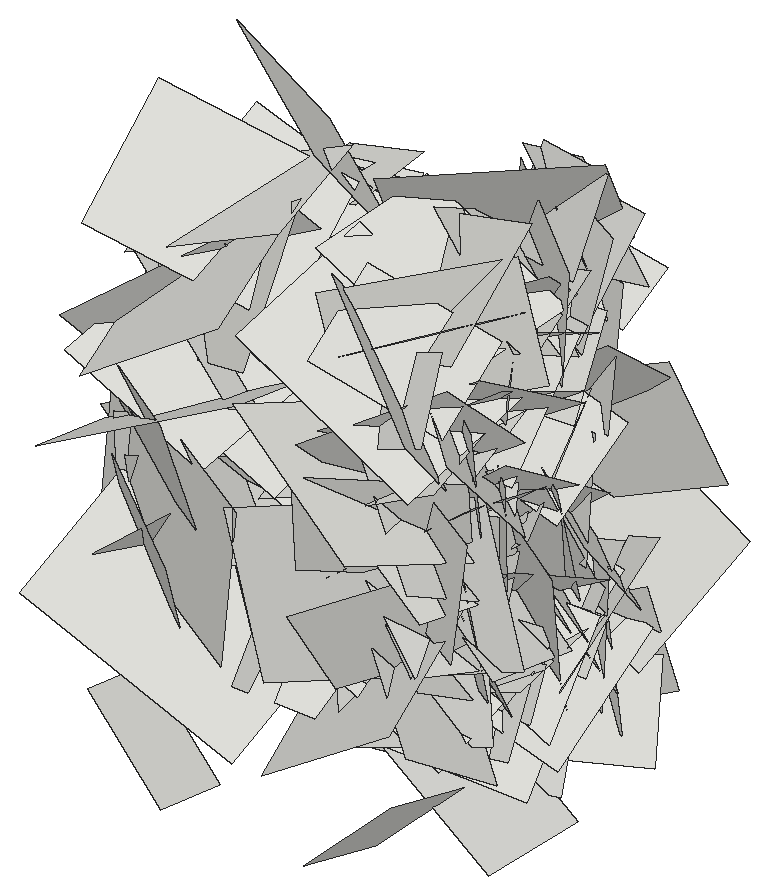
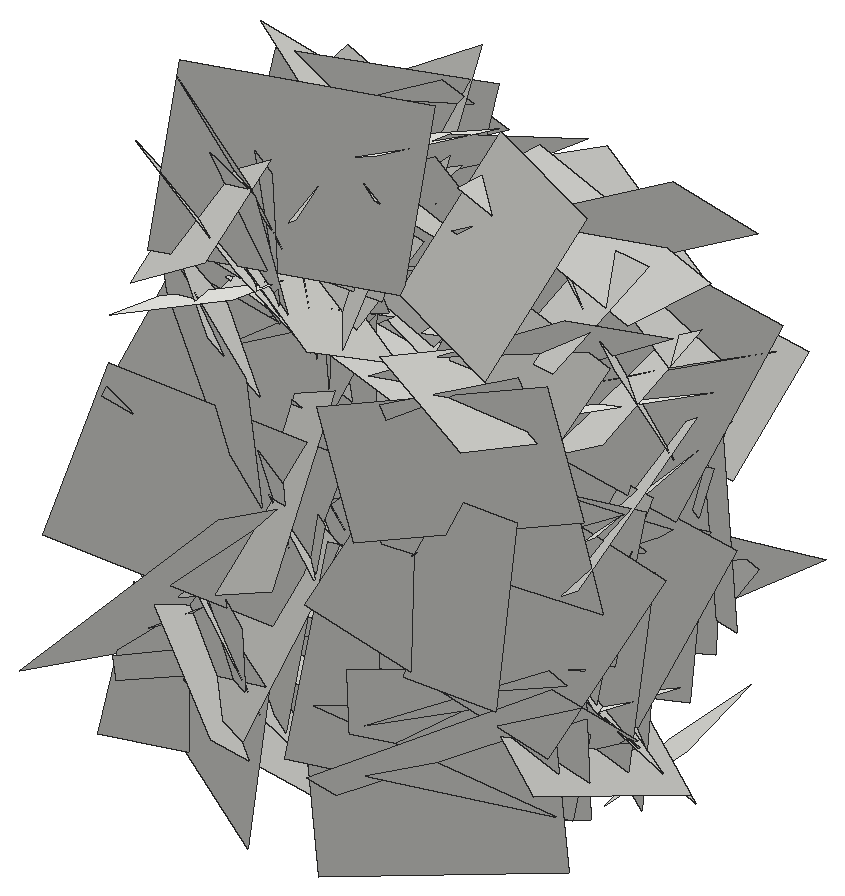
# SketchUp Ruby script. Lengths in inches.
U = 1.inch
M = Sketchup.active_model
def pt(a) = Geom::Point3d.new(a.map { |v| v * U })
def face(e, loops, mat)
  f = e.add_face(loops[0].map { |a| pt(a) })
  loops[1..].each { |l| e.add_face(l.map { |a| pt(a) }).erase! }
  f.material = f.back_material = mat if mat
  f
end
# faces: each face lists its corners as indices into pts; further lists are holes
def faces(e, pts, list, mat = nil) = list.each { |f| face(e, (f[0].is_a?(Array) ? f : [f]).map { |l| l.map { |i| pts[i] } }, mat) }
# xy, xz, yz: faces in a plane at the given z, y or x. An outline is a flat list of corners, or four numbers for a rectangle; further outlines are holes
def ring(l) = l.size == 4 ? [[l[0], l[1]], [l[2], l[1]], [l[2], l[3]], [l[0], l[3]]] : l.each_slice(2).to_a
def flat(e, list, mat, &to3) = list.each { |f| face(e, (f[0].is_a?(Array) ? f : [f]).map { |l| ring(l).map { |u, v| to3.(u, v) } }, mat) }
def xy(e, z, list, mat = nil) = flat(e, list, mat) { |x, y| [x, y, z] }
def xz(e, y, list, mat = nil) = flat(e, list, mat) { |x, z| [x, y, z] }
def yz(e, x, list, mat = nil) = flat(e, list, mat) { |y, z| [x, y, z] }
def lines(e, pts, list) = list.each { |a, b| e.add_line(pt(pts[a]), pt(pts[b])) }
# prism: a flat outline (further loops are holes) pulled along v
def prism(e, loops, v, mat = nil)
  f = face(e, loops, mat); d = Geom::Vector3d.new(v.map { |x| x * U })
  f.pushpull(f.normal.samedirection?(d) ? d.length : -d.length)
end
def box(e, o, s, mat = nil) = prism(e, [[o, [o[0] + s[0], o[1], o[2]], [o[0] + s[0], o[1] + s[1], o[2]], [o[0], o[1] + s[1], o[2]]]], [0, 0, s[2]], mat)
def at(x, y, z, deg = 0) = Geom::Transformation.translation(pt([x, y, z])) * Geom::Transformation.rotation(ORIGIN, Z_AXIS, deg.degrees)
def axes(o, x, y, z) = Geom::Transformation.new([*x, 0, *y, 0, *z, 0, *pt(o).to_a, 1])
def part(name) = M.definitions.add(name)
# library, detail: a bought-in or finely detailed component or shape, given as its bounding box
def library(name, o, s) = part(name).tap { |d| box(d.entities, o, s) }
def detail(e, o, s) = box(e.add_group.entities, o, s)
def put(e, d, t, mat = nil) = e.add_instance(d, t).tap { |i| i.material = mat if mat }
def group(e, t, mat = nil) = e.add_group.tap { |g| g.transformation = t; g.material = mat if mat }.entities
root = M.entities
c1 = part("Component\#6")
p = [[0.01,0,0],[0,3.24,4.54],[4.32,3.24,4.54],[4.33,0,0]]
faces(c1.entities,p,[[0,1,2,3]])
put(root,c1,axes([18.5,193.25,29.42],[0.0602,0.67546,-0.3863],[0.10598,-0.39045,-0.66802],[-0.81797,-0.00088,-0.11498]))
put(root,c1,axes([18.5,198.68,37.125],[-0.06347,0.58127,-0.24952],[0.07215,-0.24326,-0.58302],[-0.66662,-0.08167,-0.03935]))
put(root,c1,axes([14.53,195.125,35.61],[0.03117,0.92717,-0.40656],[-0.02653,-0.40594,-0.92757],[1.07281,-0.03698,-0.01113]))
put(root,c1,axes([18.5,200.57,36.04],[0.10099,0.61602,0.17436],[-0.1325,0.19079,-0.60575],[-0.66557,0.05549,0.14705]))
put(root,c1,axes([14.53,197.34,38.49],[0.22162,0.66132,-0.53694],[-0.02723,-0.54773,-0.68462],[0.90256,-0.17891,0.1112]))
put(root,c1,axes([14.53,198.8,27.02],[-0.0226,-0.2767,0.96977],[0.06915,0.96758,0.27751],[1.06674,-0.06859,0.00256]))
put(root,c1,axes([14.53,193.58,33.2],[0.1306,0.22319,-0.86205],[0.05382,-0.87061,-0.21815],[0.94237,0.01879,0.13193]))
put(root,c1,axes([14.53,197.85,24.73],[-0.35143,-0.52734,1.13432],[0.18025,1.14359,0.58135],[1.31365,-0.29799,0.22369]))
put(root,c1,axes([18.5,196.3,29.33],[0.09147,0.43894,-0.4809],[-0.05464,-0.47898,-0.44644],[-0.688,0.09639,-0.02848]))
put(root,c1,axes([18.5,192.39,25.48],[0.15082,-0.34829,0.66058],[0.01541,0.67363,0.35204],[-0.79143,-0.05326,0.13274]))
put(root,c1,axes([14.53,199.8,22.82],[-0.00598,0.07204,1.08492],[-0.02761,1.08461,-0.07215],[1.15221,0.02636,0.0039]))
put(root,c1,axes([18.5,194.26,19.42],[0.05867,-0.70774,0.13488],[0.12622,0.14241,0.69835],[-0.75321,-0.03127,0.12754]))
put(root,c1,axes([14.53,196.22,30.25],[-0.08073,-0.93811,0.99109],[-0.27356,0.98462,0.91216],[1.42044,0.13631,0.232]))
put(root,c1,axes([14.53,191.97,33.56],[0.08688,0.89449,0.25558],[0.12211,0.24484,-0.89383],[0.97851,-0.10998,0.08885]))
put(root,c1,axes([14.53,197.83,24.35],[-0.09568,0.96283,0.81475],[-0.1112,0.80827,-0.9668],[1.33234,0.1366,-0.02218]))
put(root,c1,axes([14.53,199.05,27.98],[0.08019,0.19915,0.92966],[0.13728,0.92174,-0.20799],[0.9984,-0.14274,-0.04607]))
put(root,c1,axes([14.53,202.95,33.21],[-0.17447,0.42234,-1.07867],[0.17991,-1.06896,-0.44444],[1.21466,0.21899,-0.08911]))
put(root,c1,axes([14.53,201.66,25.46],[-0.21728,-0.88431,0.94199],[0.03627,0.94972,0.89901],[1.36907,-0.16551,0.12568]))
put(root,c1,axes([14.53,195.04,27.27],[0.2131,0.57774,0.71728],[0.02179,0.73117,-0.59469],[0.97604,-0.14247,-0.14333]))
put(root,c1,axes([14.53,197.22,25.56],[0.17769,-0.12121,-0.94504],[0.07151,-0.95564,0.13453],[1.00742,0.08922,0.15714]))
put(root,c1,axes([14.53,192.77,37.47],[-0.01566,0.85002,0.74451],[0.07038,0.74394,-0.84805],[1.19569,-0.03266,0.05967]))
put(root,c1,axes([18.5,203.75,35.72],[0.12855,-0.35471,-0.52952],[0.05195,-0.53223,0.36775],[-0.67359,-0.10874,-0.07269]))
put(root,c1,axes([14.53,202.23,24.6],[-0.19755,-1.2824,-0.48224],[-0.04087,-0.48158,1.29554],[1.4517,-0.18807,-0.02915]))
put(root,c1,axes([14.53,200.11,31.93],[0.08158,0.26048,1.04137],[0.05734,1.04178,-0.26458],[1.13642,-0.07126,-0.06141]))
put(root,c1,axes([14.53,198.78,35.93],[0.06513,-0.64723,-0.92238],[0.00055,-0.92374,0.64822],[1.19442,0.03572,0.05]))
put(root,c1,axes([14.53,196.35,35.86],[0.06555,0.97369,0.5362],[0.0688,0.53295,-0.97527],[1.17625,-0.08544,0.02716]))
put(root,c1,axes([14.53,195.34,33.06],[0.01901,1.14103,-0.72029],[-0.19621,-0.71146,-1.13165],[1.41679,-0.11384,-0.14706]))
put(root,c1,axes([14.53,197.73,24.08],[0.06299,0.80841,0.87356],[-0.01823,0.87514,-0.8087],[1.26151,-0.02772,-0.0553]))
put(root,c1,axes([14.53,194.3,32.47],[-0.23408,0.14056,-1.33491],[0.22407,-1.33233,-0.17526],[1.40507,0.23589,-0.19445]))
put(root,c1,axes([14.53,196.04,25.17],[0.02819,1.07686,0.22249],[0.25409,0.21152,-1.05244],[1.13755,-0.07393,0.22957]))
put(root,c1,axes([14.53,193.85,32.27],[0.12737,1.17977,-0.33684],[-0.1012,-0.32843,-1.18439],[1.29659,-0.14153,-0.05935]))
put(root,c1,axes([14.53,198.24,37.08],[0.15669,-0.99926,-0.19378],[0.22295,-0.1616,0.99377],[1.05566,0.18244,-0.18112]))
put(root,c1,axes([14.53,197.21,31.46],[0.04455,0.58157,-0.95839],[0.2239,-0.94599,-0.56478],[1.16701,0.1593,0.14494]))
put(root,c1,axes([14.53,200.75,21.625],[0.14431,-0.01788,1.13958],[0.06693,1.14604,0.01044],[1.20625,-0.06145,-0.13692]))
put(root,c1,axes([14.53,198.29,23.22],[0.04433,-0.32511,1.32538],[-0.126,1.3201,0.32757],[1.44106,0.12543,-0.01213]))
put(root,c1,axes([14.53,196.35,30.1],[0.25467,1.00338,0.64071],[-0.12934,0.67094,-1.00496],[1.25528,-0.13443,-0.23354]))
put(root,c1,axes([14.53,199.72,26.12],[-0.08735,-0.8928,-1.02237],[0.07635,-1.02569,0.88989],[1.43674,0.00023,-0.10945]))
put(root,c1,axes([14.53,196.54,35.06],[0.17609,-1.11494,-0.45613],[-0.00034,-0.46049,1.12547],[1.27691,0.15363,0.0632]))
put(root,c1,axes([14.53,189.88,26.35],[0.12674,1.17916,0.69894],[-0.07675,0.70605,-1.17877],[1.45096,-0.06565,-0.1234]))
put(root,c1,axes([14.53,194.52,25.48],[0.11423,-0.20624,1.26777],[0.06819,1.2715,0.20138],[1.3598,-0.04643,-0.1166]))
put(root,c1,axes([14.53,193.84,30.46],[0.25587,-1.06575,0.3461],[0.15582,0.3811,1.07099],[1.17751,0.18115,-0.21693]))
put(root,c1,axes([14.53,199.97,41.09],[0.2759,0.65189,-0.94787],[0.07756,-0.97924,-0.65337],[1.21695,-0.08538,0.25653]))
put(root,c1,axes([14.53,200.57,23.13],[0.2198,-0.69796,1.13548],[-0.0671,1.14269,0.71395],[1.41122,0.16304,-0.1429]))
put(root,c1,axes([14.53,195.625,24.52],[0.22176,-0.47224,1.18941],[0.10161,1.2076,0.46259],[1.3527,-0.0133,-0.22974]))
put(root,c1,axes([14.53,193.54,33.12],[0.22081,1.30446,0.31828],[0.37279,0.25784,-1.28691],[1.3736,-0.27967,0.29809]))
put(root,c1,axes([28.31,193.54,33.12],[-0.22081,1.30446,0.31828],[-0.37279,0.25784,-1.28691],[-1.3736,-0.27967,0.29809]))
put(root,c1,axes([28.31,195.625,24.52],[-0.22176,-0.47224,1.18941],[-0.10161,1.2076,0.46259],[-1.3527,-0.0133,-0.22974]))
put(root,c1,axes([28.31,200.57,23.13],[-0.2198,-0.69796,1.13548],[0.0671,1.14269,0.71395],[-1.41122,0.16304,-0.1429]))
put(root,c1,axes([28.31,199.97,41.09],[-0.2759,0.65189,-0.94787],[-0.07756,-0.97924,-0.65337],[-1.21695,-0.08538,0.25653]))
put(root,c1,axes([28.31,193.84,30.46],[-0.25587,-1.06575,0.3461],[-0.15582,0.3811,1.07099],[-1.17751,0.18115,-0.21693]))
put(root,c1,axes([28.31,194.52,25.48],[-0.11423,-0.20624,1.26777],[-0.06819,1.2715,0.20138],[-1.3598,-0.04643,-0.1166]))
put(root,c1,axes([28.31,189.88,26.35],[-0.12674,1.17916,0.69894],[0.07675,0.70605,-1.17877],[-1.45096,-0.06565,-0.1234]))
put(root,c1,axes([28.31,196.54,35.06],[-0.17609,-1.11494,-0.45613],[0.00034,-0.46049,1.12547],[-1.27691,0.15363,0.0632]))
put(root,c1,axes([28.31,199.72,26.12],[0.08735,-0.8928,-1.02237],[-0.07635,-1.02569,0.88989],[-1.43674,0.00023,-0.10945]))
put(root,c1,axes([28.31,196.35,30.1],[-0.25467,1.00338,0.64071],[0.12934,0.67094,-1.00496],[-1.25528,-0.13443,-0.23354]))
put(root,c1,axes([28.31,198.29,23.22],[-0.04433,-0.32511,1.32538],[0.126,1.3201,0.32757],[-1.44106,0.12543,-0.01213]))
put(root,c1,axes([28.31,200.75,21.625],[-0.14431,-0.01788,1.13958],[-0.06693,1.14604,0.01044],[-1.20625,-0.06145,-0.13692]))
put(root,c1,axes([28.31,197.21,31.46],[-0.04455,0.58157,-0.95839],[-0.2239,-0.94599,-0.56478],[-1.16701,0.1593,0.14494]))
put(root,c1,axes([28.31,198.24,37.08],[-0.15669,-0.99926,-0.19378],[-0.22295,-0.1616,0.99377],[-1.05566,0.18244,-0.18112]))
put(root,c1,axes([28.31,193.85,32.27],[-0.12737,1.17977,-0.33684],[0.1012,-0.32843,-1.18439],[-1.29659,-0.14153,-0.05935]))
put(root,c1,axes([28.31,196.04,25.17],[-0.02819,1.07686,0.22249],[-0.25409,0.21152,-1.05244],[-1.13755,-0.07393,0.22957]))
put(root,c1,axes([28.31,194.3,32.47],[0.23408,0.14056,-1.33491],[-0.22407,-1.33233,-0.17526],[-1.40507,0.23589,-0.19445]))
put(root,c1,axes([28.31,197.73,24.08],[-0.06299,0.80841,0.87356],[0.01823,0.87514,-0.8087],[-1.26151,-0.02772,-0.0553]))
put(root,c1,axes([28.31,195.34,33.06],[-0.01901,1.14103,-0.72029],[0.19621,-0.71146,-1.13165],[-1.41679,-0.11384,-0.14706]))
put(root,c1,axes([28.31,196.35,35.86],[-0.06555,0.97369,0.5362],[-0.0688,0.53295,-0.97527],[-1.17625,-0.08544,0.02716]))
put(root,c1,axes([28.31,198.78,35.93],[-0.06513,-0.64723,-0.92238],[-0.00055,-0.92374,0.64822],[-1.19442,0.03572,0.05]))
put(root,c1,axes([28.31,200.11,31.93],[-0.08158,0.26048,1.04137],[-0.05734,1.04178,-0.26458],[-1.13642,-0.07126,-0.06141]))
put(root,c1,axes([28.31,202.23,24.6],[0.19755,-1.2824,-0.48224],[0.04087,-0.48158,1.29554],[-1.4517,-0.18807,-0.02915]))
put(root,c1,axes([24.34,203.75,35.72],[-0.12855,-0.35471,-0.52952],[-0.05195,-0.53223,0.36775],[0.67359,-0.10874,-0.07269]))
put(root,c1,axes([28.31,192.77,37.47],[0.01566,0.85002,0.74451],[-0.07038,0.74394,-0.84805],[-1.19569,-0.03266,0.05967]))
put(root,c1,axes([28.31,197.22,25.56],[-0.17769,-0.12121,-0.94504],[-0.07151,-0.95564,0.13453],[-1.00742,0.08922,0.15714]))
put(root,c1,axes([28.31,195.04,27.27],[-0.2131,0.57774,0.71728],[-0.02179,0.73117,-0.59469],[-0.97604,-0.14247,-0.14333]))
put(root,c1,axes([28.31,201.66,25.46],[0.21728,-0.88431,0.94199],[-0.03627,0.94972,0.89901],[-1.36907,-0.16551,0.12568]))
put(root,c1,axes([28.31,202.95,33.21],[0.17447,0.42234,-1.07867],[-0.17991,-1.06896,-0.44444],[-1.21466,0.21899,-0.08911]))
put(root,c1,axes([28.31,199.05,27.98],[-0.08019,0.19915,0.92966],[-0.13728,0.92174,-0.20799],[-0.9984,-0.14274,-0.04607]))
put(root,c1,axes([28.31,197.83,24.35],[0.09568,0.96283,0.81475],[0.1112,0.80827,-0.9668],[-1.33234,0.1366,-0.02218]))
put(root,c1,axes([28.31,191.97,33.56],[-0.08688,0.89449,0.25558],[-0.12211,0.24484,-0.89383],[-0.97851,-0.10998,0.08885]))
put(root,c1,axes([28.31,196.22,30.25],[0.08073,-0.93811,0.99109],[0.27356,0.98462,0.91216],[-1.42044,0.13631,0.232]))
put(root,c1,axes([24.34,194.26,19.42],[-0.05867,-0.70774,0.13488],[-0.12622,0.14241,0.69835],[0.75321,-0.03127,0.12754]))
put(root,c1,axes([28.31,199.8,22.82],[0.00598,0.07204,1.08492],[0.02761,1.08461,-0.07215],[-1.15221,0.02636,0.0039]))
put(root,c1,axes([24.34,192.39,25.48],[-0.15082,-0.34829,0.66058],[-0.01541,0.67363,0.35204],[0.79143,-0.05326,0.13274]))
put(root,c1,axes([24.34,196.3,29.33],[-0.09147,0.43894,-0.4809],[0.05464,-0.47898,-0.44644],[0.688,0.09639,-0.02848]))
put(root,c1,axes([28.31,197.85,24.73],[0.35143,-0.52734,1.13432],[-0.18025,1.14359,0.58135],[-1.31365,-0.29799,0.22369]))
put(root,c1,axes([28.31,193.58,33.2],[-0.1306,0.22319,-0.86205],[-0.05382,-0.87061,-0.21815],[-0.94237,0.01879,0.13193]))
put(root,c1,axes([28.31,198.8,27.02],[0.0226,-0.2767,0.96977],[-0.06915,0.96758,0.27751],[-1.06674,-0.06859,0.00256]))
put(root,c1,axes([28.31,197.34,38.49],[-0.22162,0.66132,-0.53694],[0.02723,-0.54773,-0.68462],[-0.90256,-0.17891,0.1112]))
put(root,c1,axes([24.34,200.57,36.04],[-0.10099,0.61602,0.17436],[0.1325,0.19079,-0.60575],[0.66557,0.05549,0.14705]))
put(root,c1,axes([28.31,195.125,35.61],[-0.03117,0.92717,-0.40656],[0.02653,-0.40594,-0.92757],[-1.07281,-0.03698,-0.01113]))
put(root,c1,axes([24.34,198.68,37.125],[0.06347,0.58127,-0.24952],[-0.07215,-0.24326,-0.58302],[0.66662,-0.08167,-0.03935]))
put(root,c1,axes([24.34,193.25,29.42],[-0.0602,0.67546,-0.3863],[-0.10598,-0.39045,-0.66802],[0.81797,-0.00088,-0.11498]))
put(root,c1,axes([24.34,194.71,36.49],[-0.01491,0.71707,-0.22931],[-0.11795,-0.22881,-0.70868],[0.78925,-0.02064,-0.11024]))
put(root,c1,axes([28.31,198.67,35.61],[0.10111,0.59855,0.78971],[-0.15679,0.79307,-0.58323],[-1.03859,-0.06146,0.16492]))
put(root,c1,axes([28.31,206.72,25.52],[0.07134,-1.27871,-0.42932],[0.37284,-0.39835,1.24159],[-1.38032,-0.17369,0.31318]))
put(root,c1,axes([28.31,196.41,37.05],[-0.02372,0.78814,-0.36288],[-0.15491,-0.36124,-0.77556],[-0.90659,0.0411,0.14202]))
put(root,c1,axes([28.31,200.08,36.17],[-0.04967,-0.3024,-0.77978],[-0.15753,-0.76557,0.30582],[-0.87244,0.15545,-0.01082]))
put(root,c1,axes([24.34,194.0625,27.88],[-0.03826,-0.32146,0.75655],[-0.14724,0.74878,0.31153],[0.85881,0.11405,0.08712]))
put(root,c1,axes([24.34,192.62,23.41],[-0.0945,0.05137,0.75973],[0.00531,0.76494,-0.05113],[0.80713,0.00098,0.08928]))
put(root,c1,axes([24.34,194.1,30.97],[-0.07757,0.18705,0.69229],[0.05179,0.69557,-0.18277],[0.75837,-0.02837,0.08329]))
put(root,c1,axes([28.31,192.76,27.5],[0.21382,-0.08753,1.03604],[-0.20559,1.03367,0.1251],[-1.08277,-0.21355,0.18084]))
put(root,c1,axes([24.34,197.11,20.7],[-0.0234,0.20043,0.60552],[0.11848,0.59772,-0.19378],[0.66563,-0.09934,0.05578]))
put(root,c1,axes([28.31,194.12,36.42],[0.16155,0.92195,-0.51802],[-0.06641,-0.51458,-0.93426],[-1.119,0.16364,-0.01934]))
put(root,c1,axes([24.34,192.68,25.51],[0.10584,0.56729,0.32604],[-0.07365,0.33715,-0.56532],[0.68964,-0.05105,-0.11041]))
put(root,c1,axes([28.31,198.72,19.65],[0.06387,-1.04135,0.05905],[0.06023,0.06234,1.04135],[-1.10396,-0.05685,0.06023]))
put(root,c1,axes([28.31,194.92,22.54],[-0.07164,-0.895,0.57486],[0.24411,0.55005,0.88344],[-1.1008,0.18023,0.15849]))
put(root,c1,axes([28.31,200.17,25.9],[-0.12286,-0.34825,-0.84521],[0.12526,-0.85054,0.33424],[-0.96086,-0.06635,0.15165]))
put(root,c1,axes([24.34,196.5,26.6],[-0.00001,0.64808,0.59207],[-0.20568,0.57742,-0.63205],[0.90746,0.13088,-0.14325]))
put(root,c1,axes([28.31,195.45,23.05],[-0.08121,0.42866,0.62692],[-0.16296,0.6083,-0.43472],[-0.78836,-0.1699,0.02528]))
put(root,c1,axes([24.34,201.07,39.9375],[-0.03161,0.68058,-0.41337],[-0.06223,-0.41441,-0.67806],[0.84176,-0.00508,-0.06565]))
put(root,c1,axes([24.34,199.74,34.07],[0.11183,-0.60219,-0.2199],[-0.02555,-0.22643,0.6085],[0.67907,0.09065,0.0591]))
put(root,c1,axes([28.31,195.7,29.31],[0.12944,0.87645,-0.3909],[-0.13192,-0.37627,-0.88251],[-1.00866,0.16168,0.06525]))
put(root,c1,axes([28.31,195.4,26.27],[-0.15303,-0.80886,0.21466],[0.08059,0.20425,0.82078],[-0.8834,0.15875,0.0377]))
put(root,c1,axes([24.34,197.17,21.41],[-0.31691,0.51794,0.91951],[-0.05422,0.94746,-0.55031],[1.11735,0.19287,0.23409]))
put(root,c1,axes([24.34,192.15,39.48],[-0.21361,0.71392,-0.72381],[-0.12034,-0.74908,-0.70723],[1.07091,0.05823,-0.22384]))
put(root,c1,axes([28.31,200.1,34.99],[-0.01875,0.74709,-0.59948],[0.09315,-0.59579,-0.74508],[-1.01106,-0.06874,-0.05753]))
put(root,c1,axes([24.34,198.57,33.25],[-0.09717,0.14422,-0.89801],[-0.11089,-0.89824,-0.13357],[0.95769,-0.08937,-0.10658]))
put(root,c1,axes([28.31,201.91,26.14],[0.02369,0.31708,-0.9382],[0.09459,-0.93526,-0.31396],[-1.04548,-0.07743,-0.04967]))
put(root,c1,axes([28.31,195.16,37.28],[-0.08536,-0.54597,-0.55526],[-0.06407,-0.55215,0.55168],[-0.82294,0.09962,0.01464]))
put(root,c1,axes([24.34,196.95,39.61],[-0.06663,0.78722,-0.39485],[-0.0883,-0.3994,-0.78302],[0.92935,0.01849,-0.10271]))
put(root,c1,axes([24.34,194.17,31.15],[-0.1572,-0.65225,0.62778],[-0.00257,0.63643,0.66066],[0.9596,-0.10514,0.10461]))
put(root,c1,axes([28.31,197.53,26.62],[-0.11622,-0.11144,-0.6986],[-0.08861,-0.69994,0.12478],[-0.74462,0.10068,0.09418]))
put(root,c1,axes([28.31,195.33,34.42],[-0.12228,0.30682,0.85432],[0.19875,0.85067,-0.2802],[-0.94146,0.13973,-0.17012]))
put(root,c1,axes([24.34,195.89,35.57],[-0.03273,-0.74668,0.19464],[0.06894,0.19158,0.74527],[0.81502,-0.04619,-0.05522]))
put(root,c1,axes([24.34,192.38,31.46],[0.05244,0.73173,-0.11131],[0.01157,-0.11227,-0.73318],[0.78447,-0.04726,0.01825]))
put(root,c1,axes([28.31,198.41,25.5],[0.14641,-1.02966,0.26735],[0.10928,0.28128,1.03005],[-1.12233,-0.10694,0.13517]))
put(root,c1,axes([28.31,198.86,35.2],[0.14047,0.16017,0.87964],[-0.13868,0.88315,-0.1411],[-0.93754,-0.10664,0.15267]))
put(root,c1,axes([24.34,193.07,33.95],[0.05953,0.85388,-0.40475],[-0.24794,-0.38029,-0.83472],[0.97048,-0.14953,-0.18843]))
put(root,c1,axes([24.34,201.02,39.48],[-0.13577,0.09163,-0.9618],[-0.05798,-0.96935,-0.08506],[1.02248,-0.0428,-0.13253]))
put(root,c1,axes([24.34,192.92,34.17],[-0.15147,-0.1521,1.01718],[-0.1212,1.02293,0.1369],[1.08344,0.09316,0.15752]))
put(root,c1,axes([28.31,191.375,35.34],[-0.1473,0.40574,0.51918],[-0.07991,0.51733,-0.42447],[-0.69387,-0.14571,-0.06134]))
put(root,c1,axes([28.31,194.18,31.13],[0.04063,-0.16003,0.87853],[0.02386,0.87924,0.15917],[-0.94627,0.0153,0.04174]))
put(root,c1,axes([24.34,202.06,39.63],[-0.00244,-0.36914,-0.6705],[0.07457,-0.66776,0.36739],[0.80789,0.06052,-0.03594]))
put(root,c1,axes([28.31,201.02,32],[0.03236,-0.79816,-0.43551],[0.07074,-0.43262,0.79753],[-0.9612,-0.0587,0.04403]))
put(root,c1,axes([28.31,199.18,25.47],[-0.11604,-0.3767,0.6399],[0.02749,0.64448,0.38383],[-0.78661,0.07809,-0.08099]))
